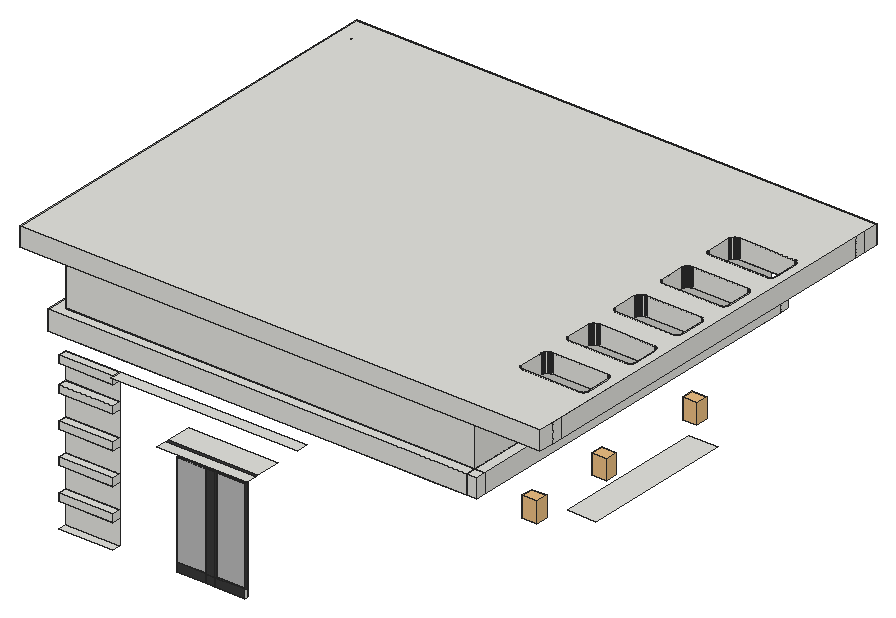
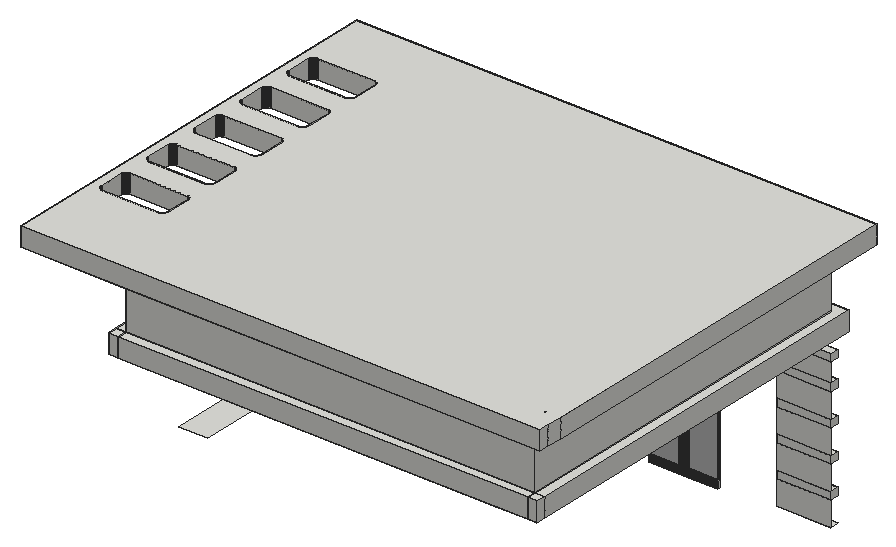
# SketchUp Ruby script. Lengths in inches.
U = 1.inch
M = Sketchup.active_model
def pt(a) = Geom::Point3d.new(a.map { |v| v * U })
def face(e, loops, mat)
  f = e.add_face(loops[0].map { |a| pt(a) })
  loops[1..].each { |l| e.add_face(l.map { |a| pt(a) }).erase! }
  f.material = f.back_material = mat if mat
  f
end
# faces: each face lists its corners as indices into pts; further lists are holes
def faces(e, pts, list, mat = nil) = list.each { |f| face(e, (f[0].is_a?(Array) ? f : [f]).map { |l| l.map { |i| pts[i] } }, mat) }
# xy, xz, yz: faces in a plane at the given z, y or x. An outline is a flat list of corners, or four numbers for a rectangle; further outlines are holes
def ring(l) = l.size == 4 ? [[l[0], l[1]], [l[2], l[1]], [l[2], l[3]], [l[0], l[3]]] : l.each_slice(2).to_a
def flat(e, list, mat, &to3) = list.each { |f| face(e, (f[0].is_a?(Array) ? f : [f]).map { |l| ring(l).map { |u, v| to3.(u, v) } }, mat) }
def xy(e, z, list, mat = nil) = flat(e, list, mat) { |x, y| [x, y, z] }
def xz(e, y, list, mat = nil) = flat(e, list, mat) { |x, z| [x, y, z] }
def yz(e, x, list, mat = nil) = flat(e, list, mat) { |y, z| [x, y, z] }
def lines(e, pts, list) = list.each { |a, b| e.add_line(pt(pts[a]), pt(pts[b])) }
# prism: a flat outline (further loops are holes) pulled along v
def prism(e, loops, v, mat = nil)
  f = face(e, loops, mat); d = Geom::Vector3d.new(v.map { |x| x * U })
  f.pushpull(f.normal.samedirection?(d) ? d.length : -d.length)
end
def box(e, o, s, mat = nil) = prism(e, [[o, [o[0] + s[0], o[1], o[2]], [o[0] + s[0], o[1] + s[1], o[2]], [o[0], o[1] + s[1], o[2]]]], [0, 0, s[2]], mat)
def at(x, y, z, deg = 0) = Geom::Transformation.translation(pt([x, y, z])) * Geom::Transformation.rotation(ORIGIN, Z_AXIS, deg.degrees)
def axes(o, x, y, z) = Geom::Transformation.new([*x, 0, *y, 0, *z, 0, *pt(o).to_a, 1])
def part(name) = M.definitions.add(name)
# library, detail: a bought-in or finely detailed component or shape, given as its bounding box
def library(name, o, s) = part(name).tap { |d| box(d.entities, o, s) }
def detail(e, o, s) = box(e.add_group.entities, o, s)
def put(e, d, t, mat = nil) = e.add_instance(d, t).tap { |i| i.material = mat if mat }
def group(e, t, mat = nil) = e.add_group.tap { |g| g.transformation = t; g.material = mat if mat }.entities
root = M.entities
M.materials.add("[Color M07]").color = [58, 58, 58]
M.materials.add("[Mirror 01]").color = [185, 185, 185]
c1 = library("Lamp Wall Outdoor 94-02",[-1.89,-4.65,-3.17],[3.78,4.65,6.35])
xy(root,309.73,[[52.28,25.1875,55.28,25.6875],[43.02,25.5,52.28,25.6875],[55.28,25.5,64.8,25.6875],[43.02,25.6875,52.28,26.1875],[52.28,25.6875,55.28,26.1875],
  [55.28,25.6875,64.8,26.1875]])
xy(root,309.73,[[43.02,25.1875,52.28,25.5],[55.28,25.1875,64.8,25.5]],"[Color M07]")
xy(root,310.73,[[7.9375,22.5,25.22,25.1875]])
xy(root,312.36,[[52.28,25.1875,55.28,25.6875],[43.02,25.5,52.28,25.6875],[43.02,25.6875,52.28,26.1875],[52.28,25.6875,55.28,26.1875],[55.28,25.6875,64.8,26.1875]])
xy(root,312.36,[[43.02,25.1875,52.28,25.5],[55.28,25.1875,64.8,25.6875]],"[Color M07]")
xy(root,318.57,[[7.9375,22.5,25.22,25.1875]])
xy(root,320.92,[[7.9375,22.5,25.22,25.1875]])
xy(root,328.75,[[7.9375,22.5,25.22,25.1875]])
xy(root,331.1,[[7.9375,22.5,25.22,25.1875]])
xy(root,336,[[128.39,73.1875,137.39,121.1875]])
xy(root,338.94,[[7.9375,22.5,25.22,25.1875]])
xy(root,341.29,[[7.9375,22.5,25.22,25.1875]])
xy(root,342.18,[[52.28,25.1875,55.28,25.6875],[43.02,25.5,52.28,25.6875],[43.02,25.6875,52.28,26.1875],[52.28,25.6875,55.28,26.1875],[55.28,25.6875,64.8,26.1875]])
xy(root,342.18,[[43.02,25.1875,52.28,25.5],[55.28,25.1875,64.8,25.6875]],"[Color M07]")
xy(root,345.39,[[39.8125,21.625,68,25.1875],[39.8125,26.1875,68,34.1875]])
xy(root,345.39,[[39.8125,25.1875,68,26.1875]],"[Color M07]")
xy(root,349.25,[[7.9375,22.5,25.22,25.1875]])
xy(root,351.6,[[7.9375,22.5,25.22,25.1875]])
xy(root,357.63,[[7.9375,22.5,25.22,25.1875]])
xy(root,359.98,[[25.22,21.625,84.16,25.1875],[7.9375,22.5,25.22,25.1875]])
xy(root,366,[[4.8125,22.0625,7.9375,25.1875],[7.9375,22.0625,16.9375,25.1875],[16.9375,22.0625,84.23,25.1875],[84.23,22.0625,84.23,24.25,86.79,24.25,86.79,25.1875,88.1,25.1875,88.1,24.25,90.66,24.25,90.66,25.1875,91.98,25.1875,91.98,24.25,94.54,24.25,94.54,25.1875,95.85,25.1875,95.85,24.25,98.41,24.25,98.41,25.1875,99.73,25.1875,99.73,24.25,102.29,24.25,102.29,25.1875,103.6,25.1875,103.6,24.25,106.16,24.25,106.16,25.1875,107.48,25.1875,107.48,24.25,110.04,24.25,110.04,25.1875,111.35,25.1875,111.35,24.25,113.91,24.25,113.91,25.1875,115.54,25.1875,115.54,24.25,118.1,24.25,118.1,25.1875,119.73,25.1875,119.73,24.25,122.29,24.25,122.29,25.1875,123.91,25.1875,123.91,24.25,126.48,24.25,126.48,25.1875,128.39,25.1875,128.39,22.0625],[128.39,22.0625,137.39,25.1875],
  [137.39,22.0625,140.51,25.1875],[84.23,24.25,86.79,25.1875],[88.1,24.25,90.66,25.1875],[91.98,24.25,94.54,25.1875],[95.85,24.25,98.41,25.1875],
  [99.73,24.25,102.29,25.1875],[103.6,24.25,106.16,25.1875],[107.48,24.25,110.04,25.1875],[111.35,24.25,113.91,25.1875],[115.54,24.25,118.1,25.1875],
  [119.73,24.25,122.29,25.1875],[123.91,24.25,126.48,25.1875],[4.8125,25.1875,7.9375,133.1875],[7.9375,25.1875,16.9375,133.1875],[16.9375,25.1875,84.23,34.1875],
  [84.23,25.1875,128.39,34.1875],[128.39,25.1875,137.39,34.1875],[137.39,25.1875,140.51,34.1875],[16.9375,34.1875,128.39,133.1875],[128.39,34.1875,137.39,133.1875],
  [137.39,34.1875,140.51,133.1875],[4.8125,133.1875,7.9375,142.1875],[7.9375,133.1875,16.9375,142.1875],[16.9375,133.1875,137.39,142.1875],[137.39,133.1875,140.51,142.1875],
  [4.8125,142.1875,7.9375,145.3125],[7.9375,142.1875,16.9375,145.3125],[16.9375,142.1875,137.39,145.3125],[137.39,142.1875,140.51,145.3125]])
xy(root,372,[[4.8125,22.0625,137.39,22.0625,137.39,25.1875,7.9375,25.1875,7.9375,142.1875,4.8125,142.1875],[137.39,22.0625,140.51,25.1875],[[7.9375,25.1875,137.39,142.1875],[16.9375,34.1875,128.39,133.1875]],[137.39,25.1875,140.51,142.1875],[16.9375,34.1875,128.39,133.1875],
  [4.8125,142.1875,7.9375,145.3125],[7.9375,142.1875,137.39,145.3125],[137.39,142.1875,140.51,145.3125]])
xy(root,390,[[0,17.25,0,142.125,4.8125,142.125,4.8125,142.1875,7.9375,142.1875,7.9375,25.1875,137.39,25.1875,137.39,142.1875,140.51,142.1875,140.51,39.73,140.52,39.54,140.56,39.36,140.62,39.1875,140.7,39.02,140.8,38.86,140.93,38.72,141.07,38.6,141.22,38.5,141.39,38.42,141.56,38.36,141.75,38.32,141.93,38.31,159.97,38.31,160.19,38.32,160.4,38.36,160.61,38.43,160.8,38.53,160.98,38.65,161.15,38.8,161.29,38.96,161.41,39.14,161.51,39.34,161.58,39.54,161.62,39.76,161.64,39.97,161.64,47.65,161.62,47.89,161.57,48.13,161.49,48.36,161.39,48.57,161.25,48.77,161.09,48.95,160.91,49.11,160.71,49.25,160.5,49.35,160.27,49.43,160.03,49.48,159.79,49.49,142.67,49.49,142.39,49.48,142.11,49.42,141.84,49.33,141.59,49.21,141.35,49.05,141.14,48.86,140.96,48.65,140.8,48.42,140.67,48.16,140.58,47.9,140.53,47.62,140.51,47.34,140.51,58.23,140.52,58.04,140.56,57.86,140.62,57.6875,140.7,57.52,140.8,57.36,140.93,57.22,141.07,57.1,141.22,57,141.39,56.92,141.56,56.86,141.75,56.82,141.93,56.81,159.97,56.81,160.19,56.82,160.4,56.86,160.61,56.93,160.8,57.03,160.98,57.15,161.15,57.3,161.29,57.46,161.41,57.64,161.51,57.84,161.58,58.04,161.62,58.26,161.64,58.47,161.64,66.15,161.62,66.39,161.57,66.63,161.49,66.86,161.39,67.07,161.25,67.27,161.09,67.45,160.91,67.61,160.71,67.75,160.5,67.85,160.27,67.93,160.03,67.98,159.79,67.99,142.67,67.99,142.39,67.98,142.11,67.92,141.84,67.83,141.59,67.71,141.35,67.55,141.14,67.36,140.96,67.15,140.8,66.92,140.67,66.66,140.58,66.4,140.53,66.12,140.51,65.84,140.51,76.73,140.52,76.54,140.56,76.36,140.62,76.1875,140.7,76.02,140.8,75.86,140.93,75.72,141.07,75.6,141.22,75.5,141.39,75.42,141.56,75.36,141.75,75.32,141.93,75.31,159.97,75.31,160.19,75.32,160.4,75.36,160.61,75.43,160.8,75.53,160.98,75.65,161.15,75.8,161.29,75.96,161.41,76.14,161.51,76.34,161.58,76.54,161.62,76.76,161.64,76.97,161.64,84.65,161.62,84.89,161.57,85.13,161.49,85.36,161.39,85.57,161.25,85.77,161.09,85.95,160.91,86.11,160.71,86.25,160.5,86.35,160.27,86.43,160.03,86.48,159.79,86.49,142.67,86.49,142.39,86.48,142.11,86.42,141.84,86.33,141.59,86.21,141.35,86.05,141.14,85.86,140.96,85.65,140.8,85.42,140.67,85.16,140.58,84.9,140.53,84.62,140.51,84.34,140.51,95.23,140.52,95.04,140.56,94.86,140.62,94.6875,140.7,94.52,140.8,94.36,140.93,94.22,141.07,94.1,141.22,94,141.39,93.92,141.56,93.86,141.75,93.82,141.93,93.81,159.97,93.81,160.19,93.82,160.4,93.86,160.61,93.93,160.8,94.03,160.98,94.15,161.15,94.3,161.29,94.46,161.41,94.64,161.51,94.84,161.58,95.04,161.62,95.26,161.64,95.47,161.64,103.15,161.62,103.39,161.57,103.63,161.49,103.86,161.39,104.07,161.25,104.27,161.09,104.45,160.91,104.61,160.71,104.75,160.5,104.85,160.27,104.93,160.03,104.98,159.79,104.99,142.67,104.99,142.39,104.98,142.11,104.92,141.84,104.83,141.59,104.71,141.35,104.55,141.14,104.36,140.96,104.15,140.8,103.92,140.67,103.66,140.58,103.4,140.53,103.12,140.51,102.84,140.51,113.73,140.52,113.54,140.56,113.36,140.62,113.1875,140.7,113.02,140.8,112.86,140.93,112.72,141.07,112.6,141.22,112.5,141.39,112.42,141.56,112.36,141.75,112.32,141.93,112.31,159.97,112.31,160.19,112.32,160.4,112.36,160.61,112.43,160.8,112.53,160.98,112.65,161.15,112.8,161.29,112.96,161.41,113.14,161.51,113.34,161.58,113.54,161.62,113.76,161.64,113.97,161.64,121.65,161.62,121.89,161.57,122.13,161.49,122.36,161.39,122.57,161.25,122.77,161.09,122.95,160.91,123.11,160.71,123.25,160.5,123.35,160.27,123.43,160.03,123.48,159.79,123.49,142.67,123.49,142.39,123.48,142.11,123.42,141.84,123.33,141.59,123.21,141.35,123.05,141.14,122.86,140.96,122.65,140.8,122.42,140.67,122.16,140.58,121.9,140.53,121.62,140.51,121.34,140.51,142.1875,164.51,142.1875,164.51,17.25],[[7.9375,25.1875,137.39,142.1875],[16.9375,34.1875,128.39,133.1875]],[0,142.125,4.8125,142.1875],[0,142.1875,4.8125,147],[4.8125,142.1875,7.9375,145.3125],
  [7.9375,142.1875,137.39,145.3125],[137.39,142.1875,140.51,145.3125],[140.51,142.1875,164.51,145.3125],[4.8125,145.3125,7.9375,150.125],[7.9375,145.3125,137.39,150.125],
  [137.39,145.3125,164.51,150.125],[0,147,4.8125,150.125]])
xy(root,396,[[[0,17.25,164.51,150.125],[141.93,112.31,141.75,112.32,141.56,112.36,141.39,112.42,141.22,112.5,141.07,112.6,140.93,112.72,140.8,112.86,140.7,113.02,140.62,113.1875,140.56,113.36,140.52,113.54,140.51,113.73,140.51,121.34,140.53,121.62,140.58,121.9,140.67,122.16,140.8,122.42,140.96,122.65,141.14,122.86,141.35,123.05,141.59,123.21,141.84,123.33,142.11,123.42,142.39,123.48,142.67,123.49,159.79,123.49,160.03,123.48,160.27,123.43,160.5,123.35,160.71,123.25,160.91,123.11,161.09,122.95,161.25,122.77,161.39,122.57,161.49,122.36,161.57,122.13,161.62,121.89,161.64,121.65,161.64,113.97,161.62,113.76,161.58,113.54,161.51,113.34,161.41,113.14,161.29,112.96,161.15,112.8,160.98,112.65,160.8,112.53,160.61,112.43,160.4,112.36,160.19,112.32,159.97,112.31],[141.93,93.81,141.75,93.82,141.56,93.86,141.39,93.92,141.22,94,141.07,94.1,140.93,94.22,140.8,94.36,140.7,94.52,140.62,94.6875,140.56,94.86,140.52,95.04,140.51,95.23,140.51,102.84,140.53,103.12,140.58,103.4,140.67,103.66,140.8,103.92,140.96,104.15,141.14,104.36,141.35,104.55,141.59,104.71,141.84,104.83,142.11,104.92,142.39,104.98,142.67,104.99,159.79,104.99,160.03,104.98,160.27,104.93,160.5,104.85,160.71,104.75,160.91,104.61,161.09,104.45,161.25,104.27,161.39,104.07,161.49,103.86,161.57,103.63,161.62,103.39,161.64,103.15,161.64,95.47,161.62,95.26,161.58,95.04,161.51,94.84,161.41,94.64,161.29,94.46,161.15,94.3,160.98,94.15,160.8,94.03,160.61,93.93,160.4,93.86,160.19,93.82,159.97,93.81],[141.93,75.31,141.75,75.32,141.56,75.36,141.39,75.42,141.22,75.5,141.07,75.6,140.93,75.72,140.8,75.86,140.7,76.02,140.62,76.1875,140.56,76.36,140.52,76.54,140.51,76.73,140.51,84.34,140.53,84.62,140.58,84.9,140.67,85.16,140.8,85.42,140.96,85.65,141.14,85.86,141.35,86.05,141.59,86.21,141.84,86.33,142.11,86.42,142.39,86.48,142.67,86.49,159.79,86.49,160.03,86.48,160.27,86.43,160.5,86.35,160.71,86.25,160.91,86.11,161.09,85.95,161.25,85.77,161.39,85.57,161.49,85.36,161.57,85.13,161.62,84.89,161.64,84.65,161.64,76.97,161.62,76.76,161.58,76.54,161.51,76.34,161.41,76.14,161.29,75.96,161.15,75.8,160.98,75.65,160.8,75.53,160.61,75.43,160.4,75.36,160.19,75.32,159.97,75.31],[141.93,56.81,141.75,56.82,141.56,56.86,141.39,56.92,141.22,57,141.07,57.1,140.93,57.22,140.8,57.36,140.7,57.52,140.62,57.6875,140.56,57.86,140.52,58.04,140.51,58.23,140.51,65.84,140.53,66.12,140.58,66.4,140.67,66.66,140.8,66.92,140.96,67.15,141.14,67.36,141.35,67.55,141.59,67.71,141.84,67.83,142.11,67.92,142.39,67.98,142.67,67.99,159.79,67.99,160.03,67.98,160.27,67.93,160.5,67.85,160.71,67.75,160.91,67.61,161.09,67.45,161.25,67.27,161.39,67.07,161.49,66.86,161.57,66.63,161.62,66.39,161.64,66.15,161.64,58.47,161.62,58.26,161.58,58.04,161.51,57.84,161.41,57.64,161.29,57.46,161.15,57.3,160.98,57.15,160.8,57.03,160.61,56.93,160.4,56.86,160.19,56.82,159.97,56.81],[141.93,38.31,141.75,38.32,141.56,38.36,141.39,38.42,141.22,38.5,141.07,38.6,140.93,38.72,140.8,38.86,140.7,39.02,140.62,39.1875,140.56,39.36,140.52,39.54,140.51,39.73,140.51,47.34,140.53,47.62,140.58,47.9,140.67,48.16,140.8,48.42,140.96,48.65,141.14,48.86,141.35,49.05,141.59,49.21,141.84,49.33,142.11,49.42,142.39,49.48,142.67,49.49,159.79,49.49,160.03,49.48,160.27,49.43,160.5,49.35,160.71,49.25,160.91,49.11,161.09,48.95,161.25,48.77,161.39,48.57,161.49,48.36,161.57,48.13,161.62,47.89,161.64,47.65,161.64,39.97,161.62,39.76,161.58,39.54,161.51,39.34,161.41,39.14,161.29,38.96,161.15,38.8,160.98,38.65,160.8,38.53,160.61,38.43,160.4,38.36,160.19,38.32,159.97,38.31]]])
xz(root,17.25,[[0,390,164.51,396]])
xz(root,22.0625,[[4.8125,366,137.39,372],[137.39,366,140.51,372]])
xz(root,22.5,[[7.9375,318.57,25.22,320.92],[7.9375,328.75,25.22,331.1],[7.9375,338.94,25.22,341.29],[7.9375,349.25,25.22,351.6],[7.9375,357.63,25.22,359.98]])
xz(root,25.1875,[[7.9375,310.73,25.22,318.57],[7.9375,318.57,25.22,320.92],[7.9375,320.92,25.22,328.75],[7.9375,328.75,25.22,331.1],[7.9375,331.1,25.22,338.94],
  [7.9375,338.94,25.22,341.29],[7.9375,341.29,25.22,349.25],[7.9375,349.25,25.22,351.6],[7.9375,351.6,25.22,357.63],[7.9375,357.63,25.22,359.98],
  [7.9375,366,137.39,372],[137.39,366,140.51,372],[7.9375,372,137.39,390]])
xz(root,25.1875,[[43.02,309.73,52.28,312.36],[52.28,309.73,55.28,312.36],[55.28,309.73,64.8,312.36],[52.28,312.36,55.28,342.18]],"[Color M07]")
xz(root,25.5,[[43.02,312.36,52.28,342.18]],"[Mirror 01]")
xz(root,25.6875,[[43.02,309.73,52.28,312.36],[52.28,309.73,55.28,312.36],[55.28,309.73,64.8,312.36],[43.02,312.36,52.28,342.18],[52.28,312.36,55.28,342.18]])
xz(root,25.6875,[[55.28,312.36,64.8,342.18]],"[Mirror 01]")
xz(root,26.1875,[[43.02,309.73,52.28,312.36],[52.28,309.73,55.28,312.36],[55.28,309.73,64.8,312.36],[52.28,312.36,55.28,342.18]],"[Color M07]")
xz(root,26.1875,[[43.02,312.36,52.28,342.18],[55.28,312.36,64.8,342.18]],"[Mirror 01]")
xz(root,34.1875,[[16.9375,372,128.39,390]])
xz(root,38.31,[[141.93,390,159.97,396]])
xz(root,49.49,[[142.67,390,159.79,396]])
xz(root,56.81,[[141.93,390,159.97,396]])
xz(root,67.99,[[142.67,390,159.79,396]])
xz(root,75.31,[[141.93,390,159.97,396]])
xz(root,86.49,[[142.67,390,159.79,396]])
xz(root,93.81,[[141.93,390,159.97,396]])
xz(root,104.99,[[142.67,390,159.79,396]])
xz(root,112.31,[[141.93,390,159.97,396]])
xz(root,123.49,[[142.67,390,159.79,396]])
xz(root,133.1875,[[16.9375,372,128.39,390]])
xz(root,142.1875,[[4.8125,366,7.9375,372],[7.9375,366,137.39,372],[137.39,366,140.51,372],[7.9375,372,137.39,390]])
xz(root,145.3125,[[4.8125,366,7.9375,372],[7.9375,366,137.39,372],[137.39,366,140.51,372]])
xz(root,150.125,[[0,390,164.51,396]])
yz(root,0,[[17.25,390,142.125,396],[142.125,390,142.1875,396],[142.1875,390,147,396],[147,390,150.125,396]])
yz(root,4.8125,[[22.0625,366,142.1875,372],[142.1875,366,145.3125,372],[142.125,390,142.1875,396]])
yz(root,7.9375,[[22.5,318.57,25.1875,320.92],[22.5,328.75,25.1875,331.1],[22.5,338.94,25.1875,341.29],[22.5,349.25,25.1875,351.6],[22.5,357.63,25.1875,359.98],
  [25.1875,366,142.1875,372],[142.1875,366,145.3125,372],[25.1875,372,142.1875,390]])
yz(root,16.9375,[[34.1875,372,133.1875,390]])
yz(root,25.22,[[22.5,318.57,25.1875,320.92],[22.5,328.75,25.1875,331.1],[22.5,338.94,25.1875,341.29],[22.5,349.25,25.1875,351.6],[22.5,357.63,25.1875,359.98]])
yz(root,43.02,[[25.1875,309.73,25.6875,312.36],[25.6875,309.73,26.1875,312.36],[25.5,312.36,25.6875,342.18],[25.6875,312.36,26.1875,342.18]])
yz(root,43.02,[[25.1875,312.36,25.5,342.18]],"[Color M07]")
yz(root,52.28,[[25.1875,309.73,25.6875,312.36],[25.6875,309.73,26.1875,312.36],[25.5,312.36,25.6875,342.18],[25.6875,312.36,26.1875,342.18]])
yz(root,52.28,[[25.1875,312.36,25.5,342.18]],"[Color M07]")
yz(root,55.28,[[25.1875,309.73,25.6875,312.36],[25.6875,309.73,26.1875,312.36],[25.6875,312.36,26.1875,342.18]])
yz(root,55.28,[[25.1875,312.36,25.6875,342.18]],"[Color M07]")
yz(root,64.8,[[25.1875,309.73,25.6875,312.36],[25.6875,309.73,26.1875,312.36],[25.6875,312.36,26.1875,342.18]])
yz(root,64.8,[[25.1875,312.36,25.6875,342.18]],"[Color M07]")
yz(root,128.39,[[34.1875,372,133.1875,390]])
yz(root,137.39,[[22.0625,366,25.1875,372],[25.1875,366,142.1875,372],[142.1875,366,145.3125,372],[25.1875,372,142.1875,390]])
yz(root,140.51,[[22.0625,366,25.1875,372],[25.1875,366,142.1875,372],[142.1875,366,145.3125,372],[39.73,390,47.34,396],[58.23,390,65.84,396],
  [76.73,390,84.34,396],[95.23,390,102.84,396],[113.73,390,121.34,396]])
yz(root,161.64,[[39.97,390,47.65,396],[58.47,390,66.15,396],[76.97,390,84.65,396],[95.47,390,103.15,396],[113.97,390,121.65,396]])
yz(root,164.51,[[17.25,390,22.0625,396],[22.0625,390,25.1875,396],[25.1875,390,142.1875,396],[142.1875,390,145.3125,396],[145.3125,390,150.125,396]])
p = [[141.56,38.36,396],[141.75,38.32,396],[141.75,38.32,390],[141.56,38.36,390],[141.93,38.31,396],[141.93,38.31,390],
  [159.97,38.31,396],[160.19,38.32,396],[160.19,38.32,390],[159.97,38.31,390],[160.4,38.36,396],[160.4,38.36,390],
  [141.22,38.5,396],[141.39,38.42,396],[141.39,38.42,390],[141.22,38.5,390],[160.61,38.43,396],[160.61,38.43,390],
  [160.8,38.53,396],[160.8,38.53,390],[141.07,38.6,396],[141.07,38.6,390],[160.98,38.65,396],[160.98,38.65,390],
  [140.93,38.72,396],[140.93,38.72,390],[140.8,38.86,396],[140.8,38.86,390],[161.15,38.8,396],[161.15,38.8,390],
  [161.29,38.96,396],[161.29,38.96,390],[140.7,39.02,396],[140.7,39.02,390],[140.62,39.1875,396],[140.62,39.1875,390],
  [161.41,39.14,396],[161.41,39.14,390],[161.51,39.34,396],[161.51,39.34,390],[140.56,39.36,396],[140.56,39.36,390],
  [161.58,39.54,396],[161.58,39.54,390],[140.52,39.54,396],[140.52,39.54,390],[140.51,39.73,396],[140.51,39.73,390],
  [161.62,39.76,396],[161.62,39.76,390],[161.64,39.97,396],[161.64,39.97,390],[140.53,47.62,396],[140.51,47.34,396],
  [140.51,47.34,390],[140.53,47.62,390],[140.58,47.9,396],[140.58,47.9,390],[161.64,47.65,396],[161.62,47.89,396],
  [161.62,47.89,390],[161.64,47.65,390],[140.67,48.16,396],[140.67,48.16,390],[161.57,48.13,396],[161.57,48.13,390],
  [161.49,48.36,396],[161.49,48.36,390],[140.8,48.42,396],[140.8,48.42,390],[140.96,48.65,396],[140.96,48.65,390],
  [161.39,48.57,396],[161.39,48.57,390],[161.25,48.77,396],[161.25,48.77,390],[141.14,48.86,396],[141.14,48.86,390],
  [161.09,48.95,396],[161.09,48.95,390],[141.35,49.05,396],[141.35,49.05,390],[141.59,49.21,396],[141.59,49.21,390],
  [160.91,49.11,396],[160.91,49.11,390],[160.71,49.25,396],[160.71,49.25,390],[141.84,49.33,396],[141.84,49.33,390],
  [160.5,49.35,396],[160.5,49.35,390],[142.11,49.42,396],[142.11,49.42,390],[142.39,49.48,396],[142.39,49.48,390],
  [160.27,49.43,396],[160.03,49.48,396],[160.03,49.48,390],[160.27,49.43,390],[142.67,49.49,396],[142.67,49.49,390],
  [159.79,49.49,396],[159.79,49.49,390],[141.56,56.86,396],[141.75,56.82,396],[141.75,56.82,390],[141.56,56.86,390],
  [141.93,56.81,396],[141.93,56.81,390],[159.97,56.81,396],[160.19,56.82,396],[160.19,56.82,390],[159.97,56.81,390],
  [160.4,56.86,396],[160.4,56.86,390],[141.22,57,396],[141.39,56.92,396],[141.39,56.92,390],[141.22,57,390],
  [160.61,56.93,396],[160.61,56.93,390],[160.8,57.03,396],[160.8,57.03,390],[141.07,57.1,396],[141.07,57.1,390],
  [160.98,57.15,396],[160.98,57.15,390],[140.93,57.22,396],[140.93,57.22,390],[140.8,57.36,396],[140.8,57.36,390],
  [161.15,57.3,396],[161.15,57.3,390],[161.29,57.46,396],[161.29,57.46,390],[140.7,57.52,396],[140.7,57.52,390],
  [140.62,57.6875,396],[140.62,57.6875,390],[161.41,57.64,396],[161.41,57.64,390],[161.51,57.84,396],[161.51,57.84,390],
  [140.56,57.86,396],[140.56,57.86,390],[161.58,58.04,396],[161.58,58.04,390],[140.52,58.04,396],[140.52,58.04,390],
  [140.51,58.23,396],[140.51,58.23,390],[161.62,58.26,396],[161.62,58.26,390],[161.64,58.47,396],[161.64,58.47,390],
  [140.53,66.12,396],[140.51,65.84,396],[140.51,65.84,390],[140.53,66.12,390],[140.58,66.4,396],[140.58,66.4,390],
  [161.64,66.15,396],[161.62,66.39,396],[161.62,66.39,390],[161.64,66.15,390],[140.67,66.66,396],[140.67,66.66,390],
  [161.57,66.63,396],[161.57,66.63,390],[161.49,66.86,396],[161.49,66.86,390],[140.8,66.92,396],[140.8,66.92,390],
  [140.96,67.15,396],[140.96,67.15,390],[161.39,67.07,396],[161.39,67.07,390],[161.25,67.27,396],[161.25,67.27,390],
  [141.14,67.36,396],[141.14,67.36,390],[161.09,67.45,396],[161.09,67.45,390],[141.35,67.55,396],[141.35,67.55,390],
  [141.59,67.71,396],[141.59,67.71,390],[160.91,67.61,396],[160.91,67.61,390],[160.71,67.75,396],[160.71,67.75,390],
  [141.84,67.83,396],[141.84,67.83,390],[160.5,67.85,396],[160.5,67.85,390],[142.11,67.92,396],[142.11,67.92,390],
  [142.39,67.98,396],[142.39,67.98,390],[160.27,67.93,396],[160.03,67.98,396],[160.03,67.98,390],[160.27,67.93,390],
  [142.67,67.99,396],[142.67,67.99,390],[159.79,67.99,396],[159.79,67.99,390],[141.56,75.36,396],[141.75,75.32,396],
  [141.75,75.32,390],[141.56,75.36,390],[141.93,75.31,396],[141.93,75.31,390],[159.97,75.31,396],[160.19,75.32,396],
  [160.19,75.32,390],[159.97,75.31,390],[160.4,75.36,396],[160.4,75.36,390],[141.22,75.5,396],[141.39,75.42,396],
  [141.39,75.42,390],[141.22,75.5,390],[160.61,75.43,396],[160.61,75.43,390],[160.8,75.53,396],[160.8,75.53,390],
  [141.07,75.6,396],[141.07,75.6,390],[160.98,75.65,396],[160.98,75.65,390],[140.93,75.72,396],[140.93,75.72,390],
  [140.8,75.86,396],[140.8,75.86,390],[161.15,75.8,396],[161.15,75.8,390],[161.29,75.96,396],[161.29,75.96,390],
  [140.7,76.02,396],[140.7,76.02,390],[140.62,76.1875,396],[140.62,76.1875,390],[161.41,76.14,396],[161.41,76.14,390],
  [161.51,76.34,396],[161.51,76.34,390],[140.56,76.36,396],[140.56,76.36,390],[161.58,76.54,396],[161.58,76.54,390],
  [140.52,76.54,396],[140.52,76.54,390],[140.51,76.73,396],[140.51,76.73,390],[161.62,76.76,396],[161.62,76.76,390],
  [161.64,76.97,396],[161.64,76.97,390],[140.53,84.62,396],[140.51,84.34,396],[140.51,84.34,390],[140.53,84.62,390],
  [140.58,84.9,396],[140.58,84.9,390],[161.64,84.65,396],[161.62,84.89,396],[161.62,84.89,390],[161.64,84.65,390],
  [140.67,85.16,396],[140.67,85.16,390],[161.57,85.13,396],[161.57,85.13,390],[161.49,85.36,396],[161.49,85.36,390],
  [140.8,85.42,396],[140.8,85.42,390],[140.96,85.65,396],[140.96,85.65,390],[161.39,85.57,396],[161.39,85.57,390],
  [161.25,85.77,396],[161.25,85.77,390],[141.14,85.86,396],[141.14,85.86,390],[161.09,85.95,396],[161.09,85.95,390],
  [141.35,86.05,396],[141.35,86.05,390],[141.59,86.21,396],[141.59,86.21,390],[160.91,86.11,396],[160.91,86.11,390],
  [160.71,86.25,396],[160.71,86.25,390],[141.84,86.33,396],[141.84,86.33,390],[160.5,86.35,396],[160.5,86.35,390],
  [142.11,86.42,396],[142.11,86.42,390],[142.39,86.48,396],[142.39,86.48,390],[160.27,86.43,396],[160.03,86.48,396],
  [160.03,86.48,390],[160.27,86.43,390],[142.67,86.49,396],[142.67,86.49,390],[159.79,86.49,396],[159.79,86.49,390],
  [141.56,93.86,396],[141.75,93.82,396],[141.75,93.82,390],[141.56,93.86,390],[141.93,93.81,396],[141.93,93.81,390],
  [159.97,93.81,396],[160.19,93.82,396],[160.19,93.82,390],[159.97,93.81,390],[160.4,93.86,396],[160.4,93.86,390],
  [141.22,94,396],[141.39,93.92,396],[141.39,93.92,390],[141.22,94,390],[160.61,93.93,396],[160.61,93.93,390],
  [160.8,94.03,396],[160.8,94.03,390],[141.07,94.1,396],[141.07,94.1,390],[160.98,94.15,396],[160.98,94.15,390],
  [140.93,94.22,396],[140.93,94.22,390],[140.8,94.36,396],[140.8,94.36,390],[161.15,94.3,396],[161.15,94.3,390],
  [161.29,94.46,396],[161.29,94.46,390],[140.7,94.52,396],[140.7,94.52,390],[140.62,94.6875,396],[140.62,94.6875,390],
  [161.41,94.64,396],[161.41,94.64,390],[161.51,94.84,396],[161.51,94.84,390],[140.56,94.86,396],[140.56,94.86,390],
  [161.58,95.04,396],[161.58,95.04,390],[140.52,95.04,396],[140.52,95.04,390],[140.51,95.23,396],[140.51,95.23,390],
  [161.62,95.26,396],[161.62,95.26,390],[161.64,95.47,396],[161.64,95.47,390],[140.53,103.12,396],[140.51,102.84,396],
  [140.51,102.84,390],[140.53,103.12,390],[140.58,103.4,396],[140.58,103.4,390],[161.64,103.15,396],[161.62,103.39,396],
  [161.62,103.39,390],[161.64,103.15,390],[140.67,103.66,396],[140.67,103.66,390],[161.57,103.63,396],[161.57,103.63,390],
  [161.49,103.86,396],[161.49,103.86,390],[140.8,103.92,396],[140.8,103.92,390],[140.96,104.15,396],[140.96,104.15,390],
  [161.39,104.07,396],[161.39,104.07,390],[161.25,104.27,396],[161.25,104.27,390],[141.14,104.36,396],[141.14,104.36,390],
  [161.09,104.45,396],[161.09,104.45,390],[141.35,104.55,396],[141.35,104.55,390],[141.59,104.71,396],[141.59,104.71,390],
  [160.91,104.61,396],[160.91,104.61,390],[160.71,104.75,396],[160.71,104.75,390],[141.84,104.83,396],[141.84,104.83,390],
  [160.5,104.85,396],[160.5,104.85,390],[142.11,104.92,396],[142.11,104.92,390],[142.39,104.98,396],[142.39,104.98,390],
  [160.27,104.93,396],[160.03,104.98,396],[160.03,104.98,390],[160.27,104.93,390],[142.67,104.99,396],[142.67,104.99,390],
  [159.79,104.99,396],[159.79,104.99,390],[141.56,112.36,396],[141.75,112.32,396],[141.75,112.32,390],[141.56,112.36,390],
  [141.93,112.31,396],[141.93,112.31,390],[159.97,112.31,396],[160.19,112.32,396],[160.19,112.32,390],[159.97,112.31,390],
  [160.4,112.36,396],[160.4,112.36,390],[141.22,112.5,396],[141.39,112.42,396],[141.39,112.42,390],[141.22,112.5,390],
  [160.61,112.43,396],[160.61,112.43,390],[160.8,112.53,396],[160.8,112.53,390],[141.07,112.6,396],[141.07,112.6,390],
  [160.98,112.65,396],[160.98,112.65,390],[140.93,112.72,396],[140.93,112.72,390],[140.8,112.86,396],[140.8,112.86,390],
  [161.15,112.8,396],[161.15,112.8,390],[161.29,112.96,396],[161.29,112.96,390],[140.7,113.02,396],[140.7,113.02,390],
  [140.62,113.1875,396],[140.62,113.1875,390],[161.41,113.14,396],[161.41,113.14,390],[161.51,113.34,396],[161.51,113.34,390],
  [140.56,113.36,396],[140.56,113.36,390],[161.58,113.54,396],[161.58,113.54,390],[140.52,113.54,396],[140.52,113.54,390],
  [140.51,113.73,396],[140.51,113.73,390],[161.62,113.76,396],[161.62,113.76,390],[161.64,113.97,396],[161.64,113.97,390],
  [140.53,121.62,396],[140.51,121.34,396],[140.51,121.34,390],[140.53,121.62,390],[140.58,121.9,396],[140.58,121.9,390],
  [161.64,121.65,396],[161.62,121.89,396],[161.62,121.89,390],[161.64,121.65,390],[140.67,122.16,396],[140.67,122.16,390],
  [161.57,122.13,396],[161.57,122.13,390],[161.49,122.36,396],[161.49,122.36,390],[140.8,122.42,396],[140.8,122.42,390],
  [140.96,122.65,396],[140.96,122.65,390],[161.39,122.57,396],[161.39,122.57,390],[161.25,122.77,396],[161.25,122.77,390],
  [141.14,122.86,396],[141.14,122.86,390],[161.09,122.95,396],[161.09,122.95,390],[141.35,123.05,396],[141.35,123.05,390],
  [141.59,123.21,396],[141.59,123.21,390],[160.91,123.11,396],[160.91,123.11,390],[160.71,123.25,396],[160.71,123.25,390],
  [141.84,123.33,396],[141.84,123.33,390],[160.5,123.35,396],[160.5,123.35,390],[142.11,123.42,396],[142.11,123.42,390],
  [142.39,123.48,396],[142.39,123.48,390],[160.27,123.43,396],[160.03,123.48,396],[160.03,123.48,390],[160.27,123.43,390],
  [142.67,123.49,396],[142.67,123.49,390],[159.79,123.49,396],[159.79,123.49,390],[7.9375,142.1875,390],[7.9375,142.1875,396],
  [140.51,25.1875,396],[140.51,25.1875,390],[140.51,142.1875,390],[140.51,142.1875,396],[140.51,22.0625,396],[140.51,22.0625,390],
  [4.8125,145.3125,390],[4.8125,145.3125,396],[4.8125,147,390],[4.8125,147,396]]
faces(root,p,[[0,1,2,3],[1,4,5,2],[6,7,8,9],[7,10,11,8],[12,13,14,15],[13,0,3,14],[10,16,17,11],[16,18,19,17],
  [20,12,15,21],[18,22,23,19],[24,20,21,25],[26,24,25,27],[22,28,29,23],[28,30,31,29],[32,26,27,33],[34,32,33,35],
  [30,36,37,31],[36,38,39,37],[40,34,35,41],[38,42,43,39],[44,40,41,45],[46,44,45,47],[42,48,49,43],[48,50,51,49],
  [52,53,54,55],[56,52,55,57],[58,59,60,61],[62,56,57,63],[59,64,65,60],[64,66,67,65],[68,62,63,69],[70,68,69,71],
  [66,72,73,67],[72,74,75,73],[76,70,71,77],[74,78,79,75],[80,76,77,81],[82,80,81,83],[78,84,85,79],[84,86,87,85],
  [88,82,83,89],[86,90,91,87],[92,88,89,93],[94,92,93,95],[96,97,98,99],[90,96,99,91],[100,94,95,101],[97,102,103,98],
  [104,105,106,107],[105,108,109,106],[110,111,112,113],[111,114,115,112],[116,117,118,119],[117,104,107,118],[114,120,121,115],[120,122,123,121],
  [124,116,119,125],[122,126,127,123],[128,124,125,129],[130,128,129,131],[126,132,133,127],[132,134,135,133],[136,130,131,137],[138,136,137,139],
  [134,140,141,135],[140,142,143,141],[144,138,139,145],[142,146,147,143],[148,144,145,149],[150,148,149,151],[146,152,153,147],[152,154,155,153],
  [156,157,158,159],[160,156,159,161],[162,163,164,165],[166,160,161,167],[163,168,169,164],[168,170,171,169],[172,166,167,173],[174,172,173,175],
  [170,176,177,171],[176,178,179,177],[180,174,175,181],[178,182,183,179],[184,180,181,185],[186,184,185,187],[182,188,189,183],[188,190,191,189],
  [192,186,187,193],[190,194,195,191],[196,192,193,197],[198,196,197,199],[200,201,202,203],[194,200,203,195],[204,198,199,205],[201,206,207,202],
  [208,209,210,211],[209,212,213,210],[214,215,216,217],[215,218,219,216],[220,221,222,223],[221,208,211,222],[218,224,225,219],[224,226,227,225],
  [228,220,223,229],[226,230,231,227],[232,228,229,233],[234,232,233,235],[230,236,237,231],[236,238,239,237],[240,234,235,241],[242,240,241,243],
  [238,244,245,239],[244,246,247,245],[248,242,243,249],[246,250,251,247],[252,248,249,253],[254,252,253,255],[250,256,257,251],[256,258,259,257],
  [260,261,262,263],[264,260,263,265],[266,267,268,269],[270,264,265,271],[267,272,273,268],[272,274,275,273],[276,270,271,277],[278,276,277,279],
  [274,280,281,275],[280,282,283,281],[284,278,279,285],[282,286,287,283],[288,284,285,289],[290,288,289,291],[286,292,293,287],[292,294,295,293],
  [296,290,291,297],[294,298,299,295],[300,296,297,301],[302,300,301,303],[304,305,306,307],[298,304,307,299],[308,302,303,309],[305,310,311,306],
  [312,313,314,315],[313,316,317,314],[318,319,320,321],[319,322,323,320],[324,325,326,327],[325,312,315,326],[322,328,329,323],[328,330,331,329],
  [332,324,327,333],[330,334,335,331],[336,332,333,337],[338,336,337,339],[334,340,341,335],[340,342,343,341],[344,338,339,345],[346,344,345,347],
  [342,348,349,343],[348,350,351,349],[352,346,347,353],[350,354,355,351],[356,352,353,357],[358,356,357,359],[354,360,361,355],[360,362,363,361],
  [364,365,366,367],[368,364,367,369],[370,371,372,373],[374,368,369,375],[371,376,377,372],[376,378,379,377],[380,374,375,381],[382,380,381,383],
  [378,384,385,379],[384,386,387,385],[388,382,383,389],[386,390,391,387],[392,388,389,393],[394,392,393,395],[390,396,397,391],[396,398,399,397],
  [400,394,395,401],[398,402,403,399],[404,400,401,405],[406,404,405,407],[408,409,410,411],[402,408,411,403],[412,406,407,413],[409,414,415,410],
  [416,417,418,419],[417,420,421,418],[422,423,424,425],[423,426,427,424],[428,429,430,431],[429,416,419,430],[426,432,433,427],[432,434,435,433],
  [436,428,431,437],[434,438,439,435],[440,436,437,441],[442,440,441,443],[438,444,445,439],[444,446,447,445],[448,442,443,449],[450,448,449,451],
  [446,452,453,447],[452,454,455,453],[456,450,451,457],[454,458,459,455],[460,456,457,461],[462,460,461,463],[458,464,465,459],[464,466,467,465],
  [468,469,470,471],[472,468,471,473],[474,475,476,477],[478,472,473,479],[475,480,481,476],[480,482,483,481],[484,478,479,485],[486,484,485,487],
  [482,488,489,483],[488,490,491,489],[492,486,487,493],[490,494,495,491],[496,492,493,497],[498,496,497,499],[494,500,501,495],[500,502,503,501],
  [504,498,499,505],[502,506,507,503],[508,504,505,509],[510,508,509,511],[512,513,514,515],[506,512,515,507],[516,510,511,517],[513,518,519,514]])
lines(root,p,[[520,521],[522,523],[524,525],[526,527],[528,529],[530,531]])
put(root,c1,at(137.39,45.83,353.05,90))
put(root,c1,at(137.39,73.39,353.05,90))
put(root,c1,at(137.39,109.27,353.05,90))
